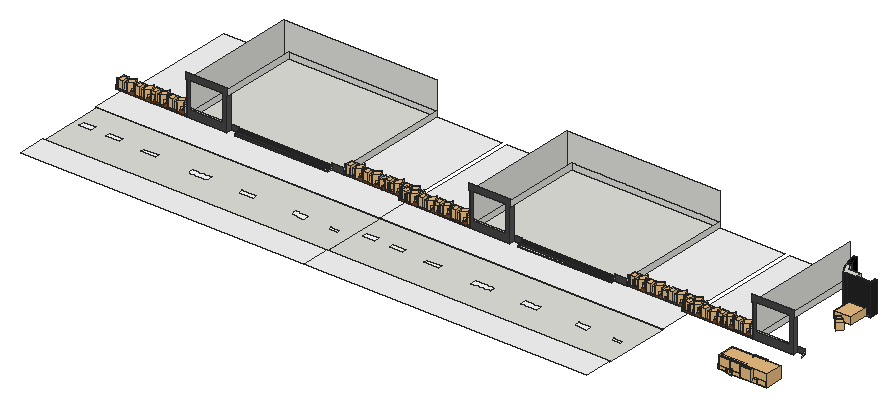
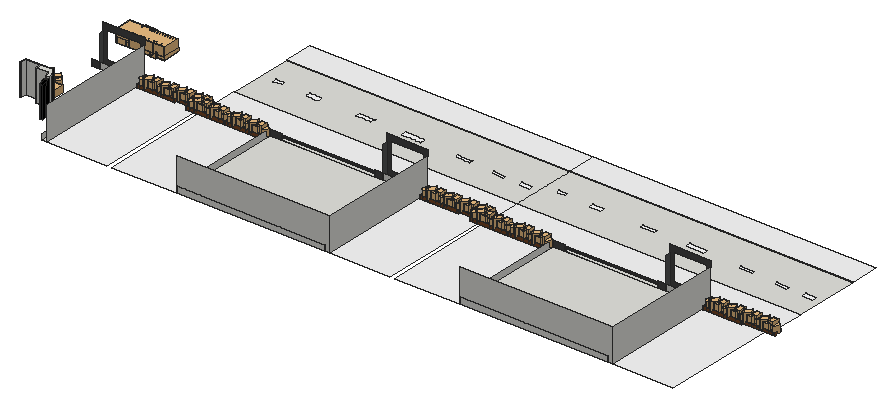
# SketchUp Ruby script. Lengths in inches.
U = 1.inch
M = Sketchup.active_model
def pt(a) = Geom::Point3d.new(a.map { |v| v * U })
def face(e, loops, mat)
  f = e.add_face(loops[0].map { |a| pt(a) })
  loops[1..].each { |l| e.add_face(l.map { |a| pt(a) }).erase! }
  f.material = f.back_material = mat if mat
  f
end
# faces: each face lists its corners as indices into pts; further lists are holes
def faces(e, pts, list, mat = nil) = list.each { |f| face(e, (f[0].is_a?(Array) ? f : [f]).map { |l| l.map { |i| pts[i] } }, mat) }
# xy, xz, yz: faces in a plane at the given z, y or x. An outline is a flat list of corners, or four numbers for a rectangle; further outlines are holes
def ring(l) = l.size == 4 ? [[l[0], l[1]], [l[2], l[1]], [l[2], l[3]], [l[0], l[3]]] : l.each_slice(2).to_a
def flat(e, list, mat, &to3) = list.each { |f| face(e, (f[0].is_a?(Array) ? f : [f]).map { |l| ring(l).map { |u, v| to3.(u, v) } }, mat) }
def xy(e, z, list, mat = nil) = flat(e, list, mat) { |x, y| [x, y, z] }
def xz(e, y, list, mat = nil) = flat(e, list, mat) { |x, z| [x, y, z] }
def yz(e, x, list, mat = nil) = flat(e, list, mat) { |y, z| [x, y, z] }
def lines(e, pts, list) = list.each { |a, b| e.add_line(pt(pts[a]), pt(pts[b])) }
# prism: a flat outline (further loops are holes) pulled along v
def prism(e, loops, v, mat = nil)
  f = face(e, loops, mat); d = Geom::Vector3d.new(v.map { |x| x * U })
  f.pushpull(f.normal.samedirection?(d) ? d.length : -d.length)
end
def box(e, o, s, mat = nil) = prism(e, [[o, [o[0] + s[0], o[1], o[2]], [o[0] + s[0], o[1] + s[1], o[2]], [o[0], o[1] + s[1], o[2]]]], [0, 0, s[2]], mat)
def at(x, y, z, deg = 0) = Geom::Transformation.translation(pt([x, y, z])) * Geom::Transformation.rotation(ORIGIN, Z_AXIS, deg.degrees)
def axes(o, x, y, z) = Geom::Transformation.new([*x, 0, *y, 0, *z, 0, *pt(o).to_a, 1])
def part(name) = M.definitions.add(name)
# library, detail: a bought-in or finely detailed component or shape, given as its bounding box
def library(name, o, s) = part(name).tap { |d| box(d.entities, o, s) }
def detail(e, o, s) = box(e.add_group.entities, o, s)
def put(e, d, t, mat = nil) = e.add_instance(d, t).tap { |i| i.material = mat if mat }
def group(e, t, mat = nil) = e.add_group.tap { |g| g.transformation = t; g.material = mat if mat }.entities
root = M.entities
M.materials.add("Aluminum_Polished").color = [83, 85, 85]
M.materials.add("Color_").color = [255, 255, 255]
M.materials.add("Material__1").color = [95, 70, 46]
M.materials.add("Sophie_Shoes2").color = [35, 35, 35]
M.materials.add("Sophie_Skirt").color = [0, 0, 0]
M.materials.add("Untitsled-1").color = [96, 91, 93]
M.materials.add("[Granite Dark Gray]").color = [69, 68, 68]
M.materials.add("[Tile Grey]").color = [249, 249, 249]
M.materials.add("[Wood Veneer 01]").color = [120, 70, 37]
M.materials.add("s500 white").color = [237, 237, 230]
M.materials.add("s600").color = [22, 22, 22]
c1 = library("Areca palm plant",[0,0,0],[49.1,36.6,54.46])
c2 = library("Group\#440",[-84.69,-90.07,-0.36],[176.51,175.13,171.4])
c3 = library("Group\#441",[-7.34,-1.2,0],[38.67,35.81,49.04])
c4 = library("Group38\#2",[14.01,28.44,-23.43],[18.58,18.32,38.89])
c5 = library("Group20\#1",[-20.81,-17.08,3.79],[39.86,39.43,37.51])
c6 = part("Group\#443")
put(c6.entities,c1,axes([76.39,-6.2,6.08],[0.56191,0.45017,0],[-0.52986,0.66137,0],[0,0,0.72]))
put(c6.entities,c1,axes([178.2,-6.2,6.08],[0.56191,0.45017,0],[-0.52986,0.66137,0],[0,0,0.72]))
put(c6.entities,c2,axes([163.5,14.93,6.05],[0.08593,-0.04961,0],[0.04961,0.08593,0],[0,0,0.10522]))
put(c6.entities,c3,axes([144.89,24.9375,8],[-0.79,0,0],[0,-0.79,0],[0,0,0.79]))
put(c6.entities,c2,axes([113.57,17.19,6.07],[0.14087,-0.08133,0],[0.08133,0.14087,0],[0,0,0.1725]))
put(c6.entities,c4,axes([235.95,-4.1,28.17],[0,0.8848,0],[-0.94674,0,0],[0,0,0.85826]))
put(c6.entities,c2,axes([190.75,14.93,6.05],[0.08593,-0.04961,0],[0.04961,0.08593,0],[0,0,0.10522]))
put(c6.entities,c2,axes([61.68,14.93,6.05],[0.08593,-0.04961,0],[0.04961,0.08593,0],[0,0,0.10522]))
put(c6.entities,c2,axes([88.93,14.93,6.05],[0.08593,-0.04961,0],[0.04961,0.08593,0],[0,0,0.10522]))
put(c6.entities,c5,axes([154.82,18.97,4.77],[-0.85,0,0],[0,-0.85,0],[0,0,0.85]))
put(c6.entities,c2,axes([41.62,14.93,6.05],[0.08593,-0.04961,0],[0.04961,0.08593,0],[0,0,0.10522]))
put(c6.entities,c2,axes([143.43,14.93,6.05],[0.08593,-0.04961,0],[0.04961,0.08593,0],[0,0,0.10522]))
put(c6.entities,c4,axes([134.14,-4.1,28.17],[0,0.8848,0],[-0.94674,0,0],[0,0,0.85826]))
g1 = group(c6.entities,at(234.8,0,0,90),"[Wood Veneer 01]")
xy(g1,0,[[0,0,6,234.8],[30,0,36,234.8]])
xy(g1,3,[[6,0,30,234.8]])
xy(g1,7,[[6,5,30,229.8]],"Material__1")
xy(g1,15,[[[0,0,36,234.8],[6,5,30,229.8]]])
xz(g1,0,[[0,0,6,0,6,3,30,3,30,0,36,0,36,15,0,15]])
xz(g1,5,[[6,7,30,15]])
xz(g1,229.8,[[6,7,30,15]])
xz(g1,234.8,[[0,0,0,15,36,15,36,0,30,0,30,3,6,3,6,0]])
yz(g1,0,[[0,0,234.8,15]])
yz(g1,6,[[0,0,234.8,3],[5,7,229.8,15]])
yz(g1,30,[[0,0,234.8,3],[5,7,229.8,15]])
yz(g1,36,[[0,0,234.8,15]])
put(c6.entities,c3,axes([43.08,24.9375,8],[-0.79,0,0],[0,-0.79,0],[0,0,0.79]))
put(c6.entities,c2,axes([11.76,17.19,6.07],[0.14087,-0.08133,0],[0.08133,0.14087,0],[0,0,0.1725]))
put(c6.entities,c5,axes([53.01,18.97,4.77],[-0.85,0,0],[0,-0.85,0],[0,0,0.85]))
put(c6.entities,c2,axes([219.01,17.19,6.07],[0.14087,-0.08133,0],[0.08133,0.14087,0],[0,0,0.1725]))
c7 = part("Untitled (5)")
xy(c7.entities,0,[[[158.81,26.5625,306.06,993.3125],[226.57,518.17,239.57,583.92],[225.28,357.51,237.28,411.51],[222.61,182.28,236.36,226.53],[239.71,931.55,251.46,972.3],[233.64,703.93,242.14,755.18],[240.05,835.03,248.8,880.53],[222.04,66.5,231.29,100.5]]])
xy(c7.entities,0,[[222.04,66.5,231.29,100.5],[222.61,182.28,236.36,226.53],[225.28,357.51,237.28,411.51],[226.57,518.17,239.57,583.92],[233.64,703.93,242.14,755.18],
  [240.05,835.03,248.8,880.53],[239.71,931.55,251.46,972.3]],"Color_")
c8 = library("Group\#638",[0,0,0],[9.48,71.95,2.68])
c9 = library("Group\#653",[0,0,0],[37.78,78.39,15.5])
c10 = library("Car wheel",[-30.53,-13.73,-29.67],[182.47,72.82,182.83])
c11 = library("Component\#55",[0,0,0],[112.42,14.7,36.85])
c12 = library("Group\#656",[0,0,0],[51.74,11.92,46.37])
c13 = library("Group\#662",[3.69,3.66,0],[191.53,68.02,49.26])
c14 = library("Group\#657",[0,0,0],[105.78,6.21,15.76])
c15 = library("Group\#639",[0,0.23,0],[177.37,78.25,22.11])
c16 = library("Group\#635",[0,0,0],[50.01,18.32,46.37])
c17 = library("Group\#86",[-0.03,0.1,-0.2],[72.93,84.1,29.53])
c18 = library("ch24 wishbone chair by Carl Hansen & Son",[0,0,0],[21.1,19.68,29.02])
c19 = library("Square table",[5.01,5.91,-0.2],[27.56,27.56,29.53])
xy(root,-20.5,[[26.62,559.875,313.69,581.125],[313.69,559.875,492.21,581.125],[527.2,559.875,939.09,581.125],[1277.25,559.875,1564.31,581.125],[1564.31,559.875,1742.84,581.125],
  [1777.83,559.875,2189.71,581.125],[2527.87,559.875,2814.94,581.125],[2814.94,559.875,2993.46,581.125],[313.69,581.125,333.44,1096.5],[333.44,581.125,990.19,1096.5],
  [1564.31,581.125,1584.06,1096.5],[1584.06,581.125,2240.81,1096.5],[2814.94,581.125,2834.69,1096.5]])
xy(root,-20.5,[[26.62,419.4375,1277.25,419.4375,1277.25,581.125,939.09,581.125,939.09,559.875,527.2,559.875,527.2,581.125,492.21,581.125,492.21,559.875,26.62,559.875],[1277.25,419.4375,2527.87,419.4375,2527.87,581.125,2189.71,581.125,2189.71,559.875,1777.83,559.875,1777.83,581.125,1742.84,581.125,1742.84,559.875,1277.25,559.875],[46.37,581.125,313.69,1096.5],[990.19,581.125,1277.25,1096.5],[1297,581.125,1564.31,1096.5],
  [2240.81,581.125,2527.87,1096.5],[2547.62,581.125,2814.94,1096.5]],"[Tile Grey]")
xy(root,-20.25,[[26.62,0,1277.25,126.25],[1277.25,0,2527.87,126.25]],"[Tile Grey]")
xy(root,-15.38,[[527.2,559.875,939.09,568.25],[1777.83,559.875,2189.71,568.25]])
xy(root,-10.73,[[527.2,568.25,939.09,575.4375],[1777.83,568.25,2189.71,575.4375]])
xy(root,-6.62,[[527.2,575.4375,939.09,578],[1777.83,575.4375,2189.71,578]])
xy(root,-3.61,[[527.2,578,939.09,580.3125],[1777.83,578,2189.71,580.3125]])
xz(root,559.875,[[[313.69,-20.5,492.21,-20.5,492.21,155.3125,310,155.3125,310,126,313.69,126],[327.6,11.5,474.41,132]],[527.2,-20.5,939.09,-15.38],[[1564.31,-20.5,1742.84,-20.5,1742.84,155.3125,1560.62,155.3125,1560.62,126,1564.31,126],[1578.23,11.5,1725.04,132]],[1777.83,-20.5,2189.71,-15.38],[[2814.94,-20.5,2993.46,-20.5,2993.46,155.3125,2811.25,155.3125,2811.25,126,2814.94,126],[2828.85,11.5,2975.66,132]]],"[Granite Dark Gray]")
xz(root,568.25,[[527.2,-15.38,939.09,-10.73],[1777.83,-15.38,2189.71,-10.73]],"[Granite Dark Gray]")
xz(root,575.4375,[[527.2,-10.73,939.09,-6.62],[1777.83,-10.73,2189.71,-6.62]],"[Granite Dark Gray]")
xz(root,578,[[527.2,-6.62,939.09,-3.61],[1777.83,-6.62,2189.71,-3.61]],"[Granite Dark Gray]")
xz(root,580.3125,[[527.2,-3.61,939.09,1.19],[1777.83,-3.61,2189.71,1.19]],"[Granite Dark Gray]")
xz(root,581.125,[[313.69,-20.5,333.44,6],[333.44,-20.5,492.21,6],[1564.31,-20.5,1584.06,6],[1584.06,-20.5,1742.84,6],[2814.94,-20.5,2834.69,6],
  [2834.69,-20.5,2993.46,6]])
xz(root,581.125,[[492.21,-20.5,527.2,6],[939.09,-20.5,990.19,6],[1742.84,-20.5,1777.83,6],[2189.71,-20.5,2240.81,6],[2993.46,-20.5,3028.45,6]],"[Granite Dark Gray]")
xz(root,1096.5,[[313.69,-20.5,313.69,126,990.19,126,990.19,6,333.44,6,333.44,-20.5],[333.44,-20.5,990.19,6],[1564.31,-20.5,1564.31,126,2240.81,126,2240.81,6,1584.06,6,1584.06,-20.5],[1584.06,-20.5,2240.81,6]])
yz(root,313.69,[[559.875,-20.5,581.125,6],[581.125,-20.5,581.125,6,559.875,6,559.875,126,1096.5,126,1096.5,-20.5]])
yz(root,333.44,[[581.125,-20.5,1096.5,6]])
yz(root,492.21,[[559.875,-20.5,581.125,120.25]],"Aluminum_Polished")
yz(root,527.2,[[559.875,-20.5,581.125,-15.38],[568.25,-15.38,581.125,-10.73],[575.4375,-10.73,581.125,-6.62],[578,-6.62,581.125,-3.61],[580.3125,-3.61,581.125,1.19]])
yz(root,939.09,[[559.875,-20.5,581.125,-15.38],[568.25,-15.38,581.125,-10.73],[575.4375,-10.73,581.125,-6.62],[578,-6.62,581.125,-3.61],[580.3125,-3.61,581.125,1.19]])
yz(root,990.19,[[581.125,-20.5,1096.5,6]])
yz(root,1564.31,[[559.875,-20.5,581.125,6],[581.125,-20.5,581.125,6,559.875,6,559.875,126,1096.5,126,1096.5,-20.5]])
yz(root,1584.06,[[581.125,-20.5,1096.5,6]])
yz(root,1742.84,[[559.875,-20.5,581.125,120.25]],"Aluminum_Polished")
yz(root,1777.83,[[559.875,-20.5,581.125,-15.38],[568.25,-15.38,581.125,-10.73],[575.4375,-10.73,581.125,-6.62],[578,-6.62,581.125,-3.61],[580.3125,-3.61,581.125,1.19]])
yz(root,2189.71,[[559.875,-20.5,581.125,-15.38],[568.25,-15.38,581.125,-10.73],[575.4375,-10.73,581.125,-6.62],[578,-6.62,581.125,-3.61],[580.3125,-3.61,581.125,1.19]])
yz(root,2240.81,[[581.125,-20.5,1096.5,6]])
yz(root,2814.94,[[559.875,-20.5,581.125,6],[581.125,-20.5,581.125,6,559.875,6,559.875,126,1096.5,126,1096.5,-20.5]])
yz(root,2834.69,[[581.125,-20.5,1096.5,6]])
yz(root,2993.46,[[559.875,-20.5,581.125,120.25]],"Aluminum_Polished")
yz(root,3028.45,[[559.875,-20.5,581.125,-15.38],[568.25,-15.38,581.125,-10.73],[575.4375,-10.73,581.125,-6.62]])
p = [[2912.71,1012.74,0],[2915.67,1002.48,0]]
lines(root,p,[[0,1]])
put(root,c6,axes([0,559.875,-20.5],[0.72468,0,0],[0,1,0],[0,0,1]))
put(root,c6,axes([140.59,566.07,-20.5],[0.72468,0,0],[0,1,0],[0,0,1]))
put(root,c7,axes([1311.52,-189.95,-24.3125],[0,1.99109,0],[-1.29,0,0],[0,0,1.29]))
put(root,c6,axes([990.19,581.125,-20.5],[0.72468,0,0],[0,1,0],[0,0,1]))
put(root,c6,axes([1160.34,581.125,-20.5],[0.72468,0,0],[0,1,0],[0,0,1]))
put(root,c6,axes([1250.625,559.875,-20.5],[0.72468,0,0],[0,1,0],[0,0,1]))
put(root,c6,axes([1391.22,566.07,-20.5],[0.72468,0,0],[0,1,0],[0,0,1]))
put(root,c7,axes([2562.14,-189.95,-24.3125],[0,1.99109,0],[-1.29,0,0],[0,0,1.29]))
put(root,c6,axes([2240.81,581.125,-20.5],[0.72468,0,0],[0,1,0],[0,0,1]))
put(root,c6,axes([2410.96,581.125,-20.5],[0.72468,0,0],[0,1,0],[0,0,1]))
put(root,c6,axes([2501.25,559.875,-20.5],[0.72468,0,0],[0,1,0],[0,0,1]))
put(root,c6,axes([2641.84,566.07,-20.5],[0.72468,0,0],[0,1,0],[0,0,1]))
g2 = group(root,at(2856.32,389.63,-1.54,-179.359))
yz(g2,0.6,[[14.08,0,32.64,0.73,14.08,0.73],[51.2,0,51.2,0.73,32.64,0.73]],"s500 white")
p = [[0,0,0.73],[0.6,14.08,0],[0.6,14.08,0.73],[0,0,0],[0.6,32.64,0.73],[0.63,32.64,0],
  [0.6,51.2,0],[0,65.27,0.73],[0.6,51.2,0.73],[0,65.27,0]]
faces(g2,p,[[0,1,2],[1,0,3],[4,1,5],[6,4,5],[6,7,8],[7,6,9]],"s500 white")
put(root,c8,at(2865.13,393.07,-0.8,-179.359),"s600")
put(root,c9,at(2890.6,396.57,-17.04,-179.359),"s600")
put(root,c10,axes([2911.28,394.62,-20.08],[-0.14272,-0.0016,0],[0.0018,-0.16111,0],[0,0,0.14273]))
put(root,c10,axes([2912.11,320.61,-20.08],[-0.14272,-0.0016,0],[-0.0018,0.16111,0],[0,0,0.14273]))
g3 = group(root,at(2896.3125,967.45,0),"Sophie_Skirt")
prism(g3,[[[16.39,45.28,0],[27.93,5.32,0],[13.08,0,0],[5.78,22.42,0],[0,45.28,0]]],[0,0,137.8])
put(root,c11,at(2968.41,398.17,-4.3,-179.359))
put(root,c11,axes([2969.31,318.34,-4.3],[-0.99994,-0.01119,0],[-0.01119,0.99994,0],[0,0,1]))
put(root,c12,axes([2956.12,385.79,-14.97],[-0.99994,-0.01119,0],[-0.01119,0.99994,0],[0,0,1]),"s600")
put(root,c12,at(2956.73,330.4375,-14.97,-179.359),"s600")
put(root,c13,axes([3071.4,317.82,-20.77],[-1.10369,-0.01236,0],[-0.01236,1.10369,0],[0,0,1.10376]))
put(root,c14,axes([3021.92,392.73,-20.06],[-0.99994,-0.01119,0],[-0.01119,0.99994,0],[0,0,1]),"s600")
put(root,c14,at(3022.68,324.98,-20.06,-179.359),"s600")
put(root,c15,at(3063.58,398.67,-20.06,-179.359),"s600")
put(root,c16,axes([3003.58,386.32,-14.97],[-0.99994,-0.01119,0],[-0.01119,0.99994,0],[0,0,1]))
put(root,c16,at(3004.2,330.97,-14.97,-179.359))
g4 = group(root,at(2914.7,894.61,0))
xy(g4,0,[[26.99,0,5.49,42.96,0,58.01,14.86,63.33,26.8,35.09,78.61,35.09,78.61,13.375,141.6,13.375,141.6,37,147.51,37,147.51,7.04,40.37,7.04,40.37,7.47]])
xy(g4,7.875,[[40.37,7.04,147.51,7.47]],"Untitsled-1")
xy(g4,137.8,[[26.99,0,40.37,7.47,147.51,7.47,147.51,37,141.6,37,141.6,13.375,78.61,13.375,78.61,35.09,26.8,35.09,14.86,63.33,0,58.01,5.49,42.96]])
xz(g4,7.04,[[40.37,0,147.51,7.875]],"Untitsled-1")
xz(g4,7.47,[[40.37,7.875,147.51,137.8]],"Sophie_Shoes2")
xz(g4,13.375,[[78.61,0,141.6,137.8]])
xz(g4,35.09,[[26.8,0,78.61,137.8]])
xz(g4,37,[[141.6,0,147.51,137.8]])
yz(g4,40.37,[[7.04,0,7.47,7.875]])
yz(g4,78.61,[[13.375,0,35.09,137.8]])
yz(g4,141.6,[[13.375,0,37,137.8]])
yz(g4,147.51,[[7.04,0,37,0,37,137.8,7.47,137.8,7.47,7.875,7.04,7.875]],"Sophie_Shoes2")
p = [[5.49,42.96,0],[26.99,0,0],[26.99,0,3.9375],[26.99,0,137.8],[5.49,42.96,137.8],[40.37,7.47,0],
  [40.37,7.47,3.9375],[26.8,35.09,0],[14.86,63.33,0],[14.86,63.33,137.8],[26.8,35.09,137.8],[0,58.01,0],
  [0,58.01,137.8],[40.37,7.47,7.875],[40.37,7.47,137.8]]
faces(g4,p,[[0,1,2,3,4],[3,2,6,13,14]],"Sophie_Shoes2")
faces(g4,p,[[5,6,2,1],[7,8,9,10],[11,0,4,12],[8,11,12,9]])
put(root,c17,at(2965.66,817.84,0))
put(root,c18,at(3005.84,777.14,0,50.338))
put(root,c19,at(3021.82,801.41,0,-129.662))
